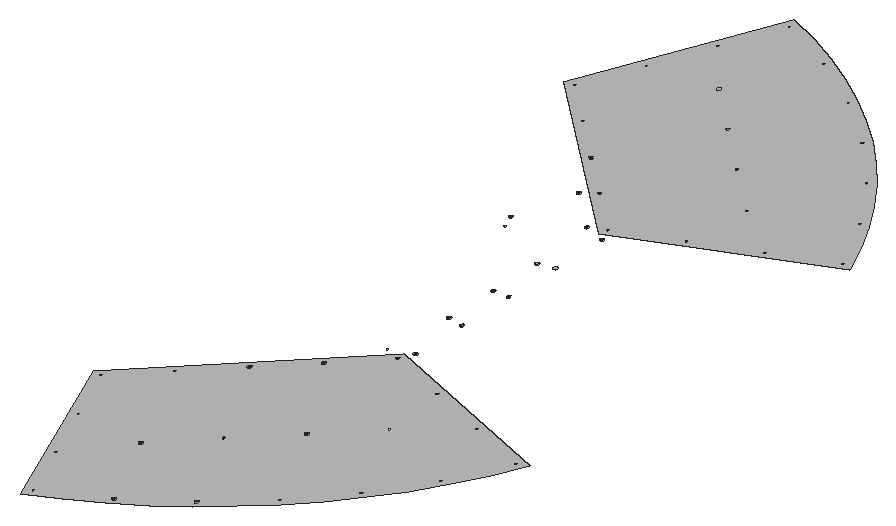
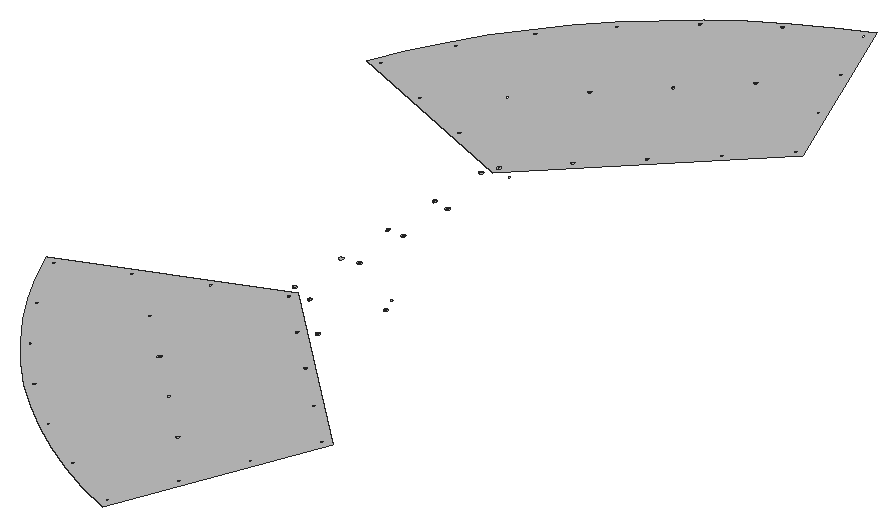
# SketchUp Ruby script. Lengths in inches.
U = 1.inch
M = Sketchup.active_model
def pt(a) = Geom::Point3d.new(a.map { |v| v * U })
def face(e, loops, mat)
  f = e.add_face(loops[0].map { |a| pt(a) })
  loops[1..].each { |l| e.add_face(l.map { |a| pt(a) }).erase! }
  f.material = f.back_material = mat if mat
  f
end
# faces: each face lists its corners as indices into pts; further lists are holes
def faces(e, pts, list, mat = nil) = list.each { |f| face(e, (f[0].is_a?(Array) ? f : [f]).map { |l| l.map { |i| pts[i] } }, mat) }
# xy, xz, yz: faces in a plane at the given z, y or x. An outline is a flat list of corners, or four numbers for a rectangle; further outlines are holes
def ring(l) = l.size == 4 ? [[l[0], l[1]], [l[2], l[1]], [l[2], l[3]], [l[0], l[3]]] : l.each_slice(2).to_a
def flat(e, list, mat, &to3) = list.each { |f| face(e, (f[0].is_a?(Array) ? f : [f]).map { |l| ring(l).map { |u, v| to3.(u, v) } }, mat) }
def xy(e, z, list, mat = nil) = flat(e, list, mat) { |x, y| [x, y, z] }
def xz(e, y, list, mat = nil) = flat(e, list, mat) { |x, z| [x, y, z] }
def yz(e, x, list, mat = nil) = flat(e, list, mat) { |y, z| [x, y, z] }
def lines(e, pts, list) = list.each { |a, b| e.add_line(pt(pts[a]), pt(pts[b])) }
# prism: a flat outline (further loops are holes) pulled along v
def prism(e, loops, v, mat = nil)
  f = face(e, loops, mat); d = Geom::Vector3d.new(v.map { |x| x * U })
  f.pushpull(f.normal.samedirection?(d) ? d.length : -d.length)
end
def box(e, o, s, mat = nil) = prism(e, [[o, [o[0] + s[0], o[1], o[2]], [o[0] + s[0], o[1] + s[1], o[2]], [o[0], o[1] + s[1], o[2]]]], [0, 0, s[2]], mat)
def at(x, y, z, deg = 0) = Geom::Transformation.translation(pt([x, y, z])) * Geom::Transformation.rotation(ORIGIN, Z_AXIS, deg.degrees)
def axes(o, x, y, z) = Geom::Transformation.new([*x, 0, *y, 0, *z, 0, *pt(o).to_a, 1])
def part(name) = M.definitions.add(name)
# library, detail: a bought-in or finely detailed component or shape, given as its bounding box
def library(name, o, s) = part(name).tap { |d| box(d.entities, o, s) }
def detail(e, o, s) = box(e.add_group.entities, o, s)
def put(e, d, t, mat = nil) = e.add_instance(d, t).tap { |i| i.material = mat if mat }
def group(e, t, mat = nil) = e.add_group.tap { |g| g.transformation = t; g.material = mat if mat }.entities
root = M.entities
M.materials.add("[Metal_Steel_Textured_White]").color = [191, 191, 191]
xy(root,3.625,[[[160.003,138.789,156.019,148.407,164.789,157.176,174.407,153.192,173.688,151.606,172.867,150.07,171.947,148.591,170.933,147.176,169.828,145.829,168.637,144.558,167.366,143.368,166.02,142.263,164.604,141.248,163.125,140.329,161.589,139.508],[162.784,154.518,162.807,154.521,162.829,154.53,162.847,154.545,162.861,154.563,162.87,154.584,162.873,154.607,162.87,154.63,162.861,154.652,162.847,154.67,162.829,154.684,162.807,154.693,162.784,154.696,162.761,154.693,162.74,154.684,162.721,154.67,162.707,154.652,162.698,154.63,162.695,154.607,162.698,154.584,162.707,154.563,162.721,154.545,162.74,154.53,162.761,154.521],[156.49,148.224,156.513,148.227,156.534,148.236,156.553,148.25,156.567,148.269,156.576,148.29,156.579,148.313,156.576,148.336,156.567,148.358,156.553,148.376,156.534,148.39,156.513,148.399,156.49,148.402,156.467,148.399,156.445,148.39,156.427,148.376,156.413,148.358,156.404,148.336,156.401,148.313,156.404,148.29,156.413,148.269,156.427,148.25,156.445,148.236,156.467,148.227],[168.355,144.751,168.378,144.755,168.399,144.763,168.418,144.778,168.432,144.796,168.441,144.817,168.444,144.84,168.441,144.863,168.432,144.885,168.418,144.903,168.399,144.917,168.378,144.926,168.355,144.929,168.332,144.926,168.31,144.917,168.292,144.903,168.278,144.885,168.269,144.863,168.266,144.84,168.269,144.817,168.278,144.796,168.292,144.778,168.31,144.763,168.332,144.755],[157.732,145.224,157.755,145.227,157.777,145.236,157.795,145.25,157.809,145.269,157.818,145.29,157.821,145.313,157.818,145.336,157.809,145.358,157.795,145.376,157.777,145.39,157.755,145.399,157.732,145.402,157.709,145.399,157.688,145.39,157.67,145.376,157.656,145.358,157.647,145.336,157.644,145.313,157.647,145.29,157.656,145.269,157.67,145.25,157.688,145.236,157.709,145.227],[158.588,150.322,158.611,150.325,158.632,150.334,158.651,150.348,158.665,150.367,158.674,150.388,158.677,150.411,158.674,150.434,158.665,150.456,158.651,150.474,158.632,150.488,158.611,150.497,158.588,150.5,158.565,150.497,158.544,150.488,158.525,150.474,158.511,150.456,158.502,150.434,158.499,150.411,158.502,150.388,158.511,150.367,158.525,150.348,158.544,150.334,158.565,150.325],[173.882,152.889,173.905,152.892,173.927,152.901,173.945,152.915,173.959,152.933,173.968,152.955,173.971,152.978,173.968,153.001,173.959,153.022,173.945,153.04,173.927,153.055,173.905,153.063,173.882,153.066,173.859,153.063,173.838,153.055,173.819,153.04,173.805,153.022,173.796,153.001,173.793,152.978,173.796,152.955,173.805,152.933,173.819,152.915,173.838,152.901,173.859,152.892],[163.155,140.72,163.178,140.723,163.2,140.732,163.218,140.746,163.232,140.764,163.241,140.786,163.244,140.809,163.241,140.832,163.232,140.853,163.218,140.871,163.2,140.886,163.178,140.894,163.155,140.897,163.132,140.894,163.111,140.886,163.093,140.871,163.078,140.853,163.07,140.832,163.066,140.809,163.07,140.786,163.078,140.764,163.093,140.746,163.111,140.732,163.132,140.723],[168.197,151.933,168.22,151.936,168.241,151.945,168.26,151.959,168.274,151.977,168.283,151.999,168.286,152.022,168.283,152.045,168.274,152.066,168.26,152.085,168.241,152.099,168.22,152.108,168.197,152.111,168.174,152.108,168.152,152.099,168.134,152.085,168.12,152.066,168.111,152.045,168.108,152.022,168.111,151.999,168.12,151.977,168.134,151.959,168.152,151.945,168.174,151.936],[170.882,154.131,170.905,154.134,170.927,154.143,170.945,154.157,170.959,154.176,170.968,154.197,170.971,154.22,170.968,154.243,170.959,154.265,170.945,154.283,170.927,154.297,170.905,154.306,170.882,154.309,170.859,154.306,170.838,154.297,170.819,154.283,170.805,154.265,170.796,154.243,170.793,154.22,170.796,154.197,170.805,154.176,170.819,154.157,170.838,154.143,170.859,154.134],[165.882,142.572,165.905,142.575,165.927,142.584,165.945,142.598,165.959,142.616,165.968,142.638,165.971,142.661,165.968,142.684,165.959,142.705,165.945,142.724,165.927,142.738,165.905,142.747,165.882,142.75,165.859,142.747,165.838,142.738,165.819,142.724,165.805,142.705,165.796,142.684,165.793,142.661,165.796,142.638,165.805,142.616,165.819,142.598,165.838,142.584,165.859,142.575],[167.882,155.374,167.905,155.377,167.927,155.386,167.945,155.4,167.959,155.418,167.968,155.44,167.971,155.463,167.968,155.486,167.959,155.507,167.945,155.526,167.927,155.54,167.905,155.549,167.882,155.552,167.859,155.549,167.838,155.54,167.819,155.526,167.805,155.507,167.796,155.486,167.793,155.463,167.796,155.44,167.805,155.418,167.819,155.4,167.838,155.386,167.859,155.377],[161.174,144.91,161.197,144.913,161.218,144.922,161.236,144.936,161.251,144.954,161.259,144.976,161.262,144.999,161.259,145.022,161.251,145.043,161.236,145.061,161.218,145.076,161.197,145.084,161.174,145.087,161.151,145.084,161.129,145.076,161.111,145.061,161.097,145.043,161.088,145.022,161.085,144.999,161.088,144.976,161.097,144.954,161.111,144.936,161.129,144.922,161.151,144.913],[165.856,149.592,165.879,149.595,165.9,149.604,165.919,149.618,165.933,149.636,165.942,149.658,165.945,149.681,165.942,149.704,165.933,149.725,165.919,149.744,165.9,149.758,165.879,149.767,165.856,149.77,165.833,149.767,165.811,149.758,165.793,149.744,165.779,149.725,165.77,149.704,165.767,149.681,165.77,149.658,165.779,149.636,165.793,149.618,165.811,149.604,165.833,149.595],[160.686,152.42,160.709,152.423,160.73,152.432,160.749,152.446,160.763,152.465,160.772,152.486,160.775,152.509,160.772,152.532,160.763,152.554,160.749,152.572,160.73,152.586,160.709,152.595,160.686,152.598,160.663,152.595,160.642,152.586,160.623,152.572,160.609,152.554,160.6,152.532,160.597,152.509,160.6,152.486,160.609,152.465,160.623,152.446,160.642,152.432,160.663,152.423],[172.387,149.951,172.41,149.954,172.431,149.963,172.45,149.977,172.464,149.995,172.473,150.017,172.476,150.04,172.473,150.063,172.464,150.084,172.45,150.103,172.431,150.117,172.41,150.126,172.387,150.129,172.364,150.126,172.342,150.117,172.324,150.103,172.31,150.084,172.301,150.063,172.298,150.04,172.301,150.017,172.31,149.995,172.324,149.977,172.342,149.963,172.364,149.954],[164.882,156.617,164.905,156.62,164.927,156.628,164.945,156.643,164.959,156.661,164.968,156.682,164.971,156.705,164.968,156.728,164.959,156.75,164.945,156.768,164.927,156.782,164.905,156.791,164.882,156.794,164.859,156.791,164.838,156.782,164.819,156.768,164.805,156.75,164.796,156.728,164.793,156.705,164.796,156.682,164.805,156.661,164.819,156.643,164.838,156.628,164.859,156.62],[158.975,142.224,158.998,142.227,159.02,142.236,159.038,142.25,159.052,142.269,159.061,142.29,159.064,142.313,159.061,142.336,159.052,142.358,159.038,142.376,159.02,142.39,158.998,142.399,158.975,142.402,158.952,142.399,158.931,142.39,158.912,142.376,158.898,142.358,158.889,142.336,158.886,142.313,158.889,142.29,158.898,142.269,158.912,142.25,158.931,142.236,158.952,142.227],[160.218,139.224,160.241,139.227,160.262,139.236,160.281,139.25,160.295,139.269,160.304,139.29,160.307,139.313,160.304,139.336,160.295,139.358,160.281,139.376,160.262,139.39,160.241,139.399,160.218,139.402,160.195,139.399,160.173,139.39,160.155,139.376,160.141,139.358,160.132,139.336,160.129,139.313,160.132,139.29,160.141,139.269,160.155,139.25,160.173,139.236,160.195,139.227],[163.515,147.251,163.538,147.254,163.559,147.263,163.577,147.277,163.592,147.295,163.6,147.317,163.604,147.34,163.6,147.363,163.592,147.384,163.577,147.402,163.559,147.417,163.538,147.425,163.515,147.429,163.492,147.425,163.47,147.417,163.452,147.402,163.4375,147.384,163.429,147.363,163.426,147.34,163.429,147.317,163.4375,147.295,163.452,147.277,163.47,147.263,163.492,147.254],[170.535,147.224,170.558,147.227,170.579,147.236,170.597,147.25,170.612,147.269,170.62,147.29,170.624,147.313,170.62,147.336,170.612,147.358,170.597,147.376,170.579,147.39,170.558,147.399,170.535,147.402,170.512,147.399,170.49,147.39,170.472,147.376,170.458,147.358,170.449,147.336,170.446,147.313,170.449,147.29,170.458,147.269,170.472,147.25,170.49,147.236,170.512,147.227]],[[163.155,140.72,163.132,140.723,163.111,140.732,163.093,140.746,163.078,140.764,163.07,140.786,163.066,140.809,163.07,140.832,163.078,140.853,163.093,140.871,163.111,140.886,163.132,140.894,163.155,140.897,163.178,140.894,163.2,140.886,163.218,140.871,163.232,140.853,163.241,140.832,163.244,140.809,163.241,140.786,163.232,140.764,163.218,140.746,163.2,140.732,163.178,140.723],[163.155,140.721,163.178,140.724,163.199,140.732,163.218,140.746,163.232,140.765,163.24,140.786,163.243,140.809,163.24,140.831,163.232,140.852,163.218,140.871,163.199,140.885,163.178,140.893,163.155,140.896,163.133,140.893,163.111,140.885,163.093,140.871,163.079,140.852,163.07,140.831,163.067,140.809,163.07,140.786,163.079,140.765,163.093,140.746,163.111,140.732,163.133,140.724]],[[163.155,140.721,163.133,140.724,163.111,140.732,163.093,140.746,163.079,140.765,163.07,140.786,163.067,140.809,163.07,140.831,163.079,140.852,163.093,140.871,163.111,140.885,163.133,140.893,163.155,140.896,163.178,140.893,163.199,140.885,163.218,140.871,163.232,140.852,163.24,140.831,163.243,140.809,163.24,140.786,163.232,140.765,163.218,140.746,163.199,140.732,163.178,140.724],[163.155,140.772,163.165,140.773,163.174,140.777,163.181,140.783,163.187,140.79,163.191,140.799,163.192,140.809,163.191,140.818,163.187,140.827,163.181,140.834,163.174,140.84,163.165,140.844,163.155,140.845,163.146,140.844,163.137,140.84,163.13,140.834,163.124,140.827,163.12,140.818,163.119,140.809,163.12,140.799,163.124,140.79,163.13,140.783,163.137,140.777,163.146,140.773]],[163.15,140.789,163.145,140.791,163.141,140.794,163.138,140.799,163.136,140.803,163.135,140.809,163.136,140.814,163.138,140.819,163.141,140.823,163.145,140.826,163.15,140.828,163.161,140.828,163.165,140.826,163.169,140.823,163.173,140.819,163.175,140.814,163.175,140.803,163.173,140.799,163.169,140.794,163.165,140.791,163.161,140.789],[[165.882,142.572,165.859,142.575,165.838,142.584,165.819,142.598,165.805,142.616,165.796,142.638,165.793,142.661,165.796,142.684,165.805,142.705,165.819,142.724,165.838,142.738,165.859,142.747,165.882,142.75,165.905,142.747,165.927,142.738,165.945,142.724,165.959,142.705,165.968,142.684,165.971,142.661,165.968,142.638,165.959,142.616,165.945,142.598,165.927,142.584,165.905,142.575],[165.882,142.573,165.905,142.576,165.926,142.585,165.944,142.599,165.958,142.617,165.967,142.638,165.97,142.661,165.967,142.683,165.958,142.705,165.944,142.723,165.926,142.737,165.905,142.746,165.882,142.749,165.859,142.746,165.838,142.737,165.82,142.723,165.806,142.705,165.797,142.683,165.794,142.661,165.797,142.638,165.806,142.617,165.82,142.599,165.838,142.585,165.859,142.576]],
  [[165.882,142.573,165.859,142.576,165.838,142.585,165.82,142.599,165.806,142.617,165.797,142.638,165.794,142.661,165.797,142.683,165.806,142.705,165.82,142.723,165.838,142.737,165.859,142.746,165.882,142.749,165.905,142.746,165.926,142.737,165.944,142.723,165.958,142.705,165.967,142.683,165.97,142.661,165.967,142.638,165.958,142.617,165.944,142.599,165.926,142.585,165.905,142.576],[165.882,142.624,165.892,142.625,165.9,142.629,165.908,142.635,165.914,142.642,165.917,142.651,165.919,142.661,165.917,142.67,165.914,142.679,165.908,142.687,165.9,142.692,165.892,142.696,165.882,142.697,165.873,142.696,165.864,142.692,165.856,142.687,165.85,142.679,165.847,142.67,165.846,142.661,165.847,142.651,165.85,142.642,165.856,142.635,165.864,142.629,165.873,142.625]],[[161.174,144.91,161.151,144.913,161.129,144.922,161.111,144.936,161.097,144.954,161.088,144.976,161.085,144.999,161.088,145.022,161.097,145.043,161.111,145.061,161.129,145.076,161.151,145.084,161.174,145.087,161.197,145.084,161.218,145.076,161.236,145.061,161.251,145.043,161.259,145.022,161.262,144.999,161.259,144.976,161.251,144.954,161.236,144.936,161.218,144.922,161.197,144.913],[161.174,144.911,161.196,144.914,161.218,144.922,161.236,144.936,161.25,144.955,161.258,144.976,161.261,144.999,161.258,145.021,161.25,145.043,161.236,145.061,161.218,145.075,161.196,145.083,161.174,145.086,161.151,145.083,161.13,145.075,161.111,145.061,161.097,145.043,161.089,145.021,161.086,144.999,161.089,144.976,161.097,144.955,161.111,144.936,161.13,144.922,161.151,144.914]],[[163.515,147.251,163.492,147.254,163.47,147.263,163.452,147.277,163.4375,147.295,163.429,147.317,163.426,147.34,163.429,147.363,163.4375,147.384,163.452,147.402,163.47,147.417,163.492,147.425,163.515,147.429,163.538,147.425,163.559,147.417,163.577,147.402,163.592,147.384,163.6,147.363,163.604,147.34,163.6,147.317,163.592,147.295,163.577,147.277,163.559,147.263,163.538,147.254],[163.515,147.252,163.537,147.255,163.559,147.263,163.577,147.277,163.591,147.296,163.6,147.317,163.603,147.34,163.6,147.362,163.591,147.384,163.577,147.402,163.559,147.416,163.537,147.425,163.515,147.428,163.492,147.425,163.471,147.416,163.452,147.402,163.438,147.384,163.43,147.362,163.427,147.34,163.43,147.317,163.438,147.296,163.452,147.277,163.471,147.263,163.492,147.255]],[[163.515,147.303,163.505,147.304,163.496,147.308,163.489,147.314,163.483,147.321,163.479,147.33,163.478,147.34,163.479,147.349,163.483,147.358,163.489,147.365,163.496,147.371,163.505,147.375,163.515,147.376,163.524,147.375,163.533,147.371,163.541,147.365,163.546,147.358,163.55,147.349,163.551,147.34,163.55,147.33,163.546,147.321,163.541,147.314,163.533,147.308,163.524,147.304],[163.509,147.32,163.52,147.32,163.525,147.322,163.529,147.326,163.532,147.33,163.534,147.334,163.535,147.34,163.534,147.345,163.532,147.35,163.529,147.354,163.525,147.357,163.52,147.359,163.515,147.36,163.509,147.359,163.505,147.357,163.501,147.354,163.497,147.35,163.495,147.345,163.495,147.334,163.497,147.33,163.505,147.322]],[163.509,147.32,163.505,147.322,163.497,147.33,163.495,147.334,163.495,147.345,163.497,147.35,163.501,147.354,163.505,147.357,163.509,147.359,163.515,147.36,163.52,147.359,163.525,147.357,163.529,147.354,163.532,147.35,163.534,147.345,163.535,147.34,163.534,147.334,163.532,147.33,163.529,147.326,163.525,147.322,163.52,147.32],
  [[165.856,149.592,165.833,149.595,165.811,149.604,165.793,149.618,165.779,149.636,165.77,149.658,165.767,149.681,165.77,149.704,165.779,149.725,165.793,149.744,165.811,149.758,165.833,149.767,165.856,149.77,165.879,149.767,165.9,149.758,165.919,149.744,165.933,149.725,165.942,149.704,165.945,149.681,165.942,149.658,165.933,149.636,165.919,149.618,165.9,149.604,165.879,149.595],[165.856,149.593,165.878,149.596,165.9,149.605,165.918,149.619,165.932,149.637,165.941,149.658,165.944,149.681,165.941,149.703,165.932,149.725,165.918,149.743,165.9,149.757,165.878,149.766,165.856,149.769,165.833,149.766,165.812,149.757,165.794,149.743,165.78,149.725,165.771,149.703,165.768,149.681,165.771,149.658,165.78,149.637,165.794,149.619,165.812,149.605,165.833,149.596]],[[160.686,152.42,160.663,152.423,160.642,152.432,160.623,152.446,160.609,152.465,160.6,152.486,160.597,152.509,160.6,152.532,160.609,152.554,160.623,152.572,160.642,152.586,160.663,152.595,160.686,152.598,160.709,152.595,160.73,152.586,160.749,152.572,160.763,152.554,160.772,152.532,160.775,152.509,160.772,152.486,160.763,152.465,160.749,152.446,160.73,152.432,160.709,152.423],[160.686,152.421,160.709,152.424,160.73,152.433,160.748,152.447,160.762,152.465,160.771,152.487,160.774,152.509,160.771,152.532,160.762,152.553,160.748,152.571,160.73,152.585,160.709,152.594,160.686,152.597,160.663,152.594,160.642,152.585,160.624,152.571,160.61,152.553,160.601,152.532,160.598,152.509,160.601,152.487,160.61,152.465,160.624,152.447,160.642,152.433,160.663,152.424]],[[160.686,152.473,160.677,152.474,160.668,152.478,160.66,152.483,160.654,152.491,160.651,152.5,160.649,152.509,160.651,152.519,160.654,152.528,160.66,152.535,160.668,152.541,160.677,152.545,160.686,152.546,160.696,152.545,160.704,152.541,160.712,152.535,160.718,152.528,160.721,152.519,160.723,152.509,160.721,152.5,160.718,152.491,160.712,152.483,160.704,152.478,160.696,152.474],[160.686,152.489,160.691,152.49,160.696,152.492,160.7,152.495,160.703,152.499,160.705,152.504,160.706,152.509,160.705,152.514,160.703,152.519,160.7,152.523,160.696,152.527,160.691,152.529,160.681,152.529,160.676,152.527,160.672,152.523,160.669,152.519,160.667,152.514,160.666,152.509,160.667,152.504,160.669,152.499,160.672,152.495,160.676,152.492,160.681,152.49]],[160.686,152.489,160.681,152.49,160.676,152.492,160.672,152.495,160.669,152.499,160.667,152.504,160.666,152.509,160.667,152.514,160.669,152.519,160.672,152.523,160.676,152.527,160.681,152.529,160.691,152.529,160.696,152.527,160.7,152.523,160.703,152.519,160.705,152.514,160.706,152.509,160.705,152.504,160.703,152.499,160.7,152.495,160.696,152.492,160.691,152.49],[[162.784,154.518,162.761,154.521,162.74,154.53,162.721,154.545,162.707,154.563,162.698,154.584,162.695,154.607,162.698,154.63,162.707,154.652,162.721,154.67,162.74,154.684,162.761,154.693,162.784,154.696,162.807,154.693,162.829,154.684,162.847,154.67,162.861,154.652,162.87,154.63,162.873,154.607,162.87,154.584,162.861,154.563,162.847,154.545,162.829,154.53,162.807,154.521],[162.784,154.519,162.807,154.522,162.828,154.531,162.846,154.545,162.86,154.563,162.869,154.585,162.872,154.607,162.869,154.63,162.86,154.651,162.846,154.67,162.828,154.684,162.807,154.692,162.784,154.695,162.761,154.692,162.74,154.684,162.722,154.67,162.708,154.651,162.699,154.63,162.696,154.607,162.699,154.585,162.708,154.563,162.722,154.545,162.74,154.531,162.761,154.522]],
  [[162.784,154.519,162.761,154.522,162.74,154.531,162.722,154.545,162.708,154.563,162.699,154.585,162.696,154.607,162.699,154.63,162.708,154.651,162.722,154.67,162.74,154.684,162.761,154.692,162.784,154.695,162.807,154.692,162.828,154.684,162.846,154.67,162.86,154.651,162.869,154.63,162.872,154.607,162.869,154.585,162.86,154.563,162.846,154.545,162.828,154.531,162.807,154.522],[162.784,154.571,162.794,154.572,162.802,154.576,162.81,154.581,162.816,154.589,162.819,154.598,162.821,154.607,162.819,154.617,162.816,154.626,162.81,154.633,162.802,154.639,162.794,154.643,162.784,154.644,162.775,154.643,162.766,154.639,162.758,154.633,162.752,154.626,162.749,154.617,162.748,154.607,162.749,154.598,162.752,154.589,162.758,154.581,162.766,154.576,162.775,154.572]],[[167.882,155.426,167.873,155.427,167.864,155.431,167.856,155.437,167.851,155.445,167.847,155.453,167.846,155.463,167.847,155.472,167.851,155.481,167.856,155.489,167.864,155.495,167.873,155.498,167.882,155.499,167.892,155.498,167.901,155.495,167.908,155.489,167.914,155.481,167.918,155.472,167.919,155.463,167.918,155.453,167.914,155.445,167.908,155.437,167.901,155.431,167.892,155.427],[167.882,155.443,167.887,155.444,167.892,155.446,167.896,155.449,167.899,155.453,167.901,155.458,167.902,155.463,167.901,155.468,167.899,155.473,167.896,155.477,167.892,155.48,167.887,155.482,167.882,155.483,167.877,155.482,167.872,155.48,167.868,155.477,167.865,155.473,167.863,155.468,167.862,155.463,167.863,155.458,167.865,155.453,167.868,155.449,167.872,155.446,167.877,155.444]],[167.882,155.443,167.877,155.444,167.872,155.446,167.868,155.449,167.865,155.453,167.863,155.458,167.862,155.463,167.863,155.468,167.865,155.473,167.868,155.477,167.872,155.48,167.877,155.482,167.882,155.483,167.887,155.482,167.892,155.48,167.896,155.477,167.899,155.473,167.901,155.468,167.902,155.463,167.901,155.458,167.899,155.453,167.896,155.449,167.892,155.446,167.887,155.444],[[164.882,156.618,164.859,156.621,164.838,156.629,164.82,156.643,164.806,156.661,164.797,156.683,164.794,156.705,164.797,156.728,164.806,156.749,164.82,156.768,164.838,156.782,164.859,156.79,164.882,156.793,164.905,156.79,164.926,156.782,164.944,156.768,164.958,156.749,164.967,156.728,164.97,156.705,164.967,156.683,164.958,156.661,164.944,156.643,164.926,156.629,164.905,156.621],[164.882,156.669,164.892,156.67,164.901,156.674,164.908,156.68,164.914,156.687,164.918,156.696,164.919,156.705,164.918,156.715,164.914,156.724,164.908,156.731,164.901,156.737,164.892,156.741,164.882,156.742,164.873,156.741,164.864,156.737,164.856,156.731,164.851,156.724,164.847,156.715,164.846,156.705,164.847,156.696,164.851,156.687,164.856,156.68,164.864,156.674,164.873,156.67]],[164.882,156.685,164.877,156.686,164.872,156.688,164.868,156.691,164.865,156.695,164.863,156.7,164.862,156.705,164.863,156.711,164.865,156.715,164.868,156.72,164.872,156.723,164.877,156.725,164.887,156.725,164.892,156.723,164.896,156.72,164.9,156.715,164.902,156.711,164.902,156.7,164.9,156.695,164.896,156.691,164.892,156.688,164.887,156.686],
  [164.084,157.016,164.079,157.017,164.074,157.019,164.07,157.022,164.067,157.026,164.065,157.031,164.064,157.036,164.065,157.041,164.067,157.046,164.07,157.05,164.074,157.053,164.079,157.055,164.084,157.056,164.089,157.055,164.094,157.053,164.098,157.05,164.101,157.046,164.103,157.041,164.104,157.036,164.103,157.031,164.101,157.026,164.098,157.022,164.094,157.019,164.089,157.017],[[165.188,157.354,165.165,157.357,165.143,157.366,165.125,157.38,165.111,157.399,165.102,157.42,165.099,157.443,165.102,157.466,165.111,157.488,165.125,157.506,165.143,157.52,165.165,157.529,165.188,157.532,165.211,157.529,165.232,157.52,165.251,157.506,165.265,157.488,165.274,157.466,165.277,157.443,165.274,157.42,165.265,157.399,165.251,157.38,165.232,157.366,165.211,157.357],[165.188,157.355,165.211,157.358,165.232,157.367,165.25,157.381,165.264,157.399,165.273,157.42,165.276,157.443,165.273,157.466,165.264,157.487,165.25,157.505,165.232,157.519,165.211,157.528,165.188,157.531,165.165,157.528,165.144,157.519,165.126,157.505,165.112,157.487,165.103,157.466,165.1,157.443,165.103,157.42,165.112,157.399,165.126,157.381,165.144,157.367,165.165,157.358]],[[165.188,157.355,165.165,157.358,165.144,157.367,165.126,157.381,165.112,157.399,165.103,157.42,165.1,157.443,165.103,157.466,165.112,157.487,165.126,157.505,165.144,157.519,165.165,157.528,165.188,157.531,165.211,157.528,165.232,157.519,165.25,157.505,165.264,157.487,165.273,157.466,165.276,157.443,165.273,157.42,165.264,157.399,165.25,157.381,165.232,157.367,165.211,157.358],[165.188,157.407,165.197,157.408,165.206,157.411,165.214,157.417,165.219,157.425,165.223,157.434,165.224,157.443,165.223,157.453,165.219,157.461,165.214,157.469,165.206,157.475,165.197,157.478,165.188,157.48,165.178,157.478,165.169,157.475,165.162,157.469,165.156,157.461,165.152,157.453,165.151,157.443,165.152,157.434,165.156,157.425,165.162,157.417,165.169,157.411,165.178,157.408]],[[165.188,160.321,165.165,160.324,165.143,160.333,165.125,160.347,165.111,160.366,165.102,160.387,165.099,160.41,165.102,160.433,165.111,160.455,165.125,160.473,165.143,160.487,165.165,160.496,165.188,160.499,165.211,160.496,165.232,160.487,165.251,160.473,165.265,160.455,165.274,160.433,165.277,160.41,165.274,160.387,165.265,160.366,165.251,160.347,165.232,160.333,165.211,160.324],[165.188,160.322,165.211,160.325,165.232,160.334,165.25,160.348,165.264,160.366,165.273,160.388,165.276,160.41,165.273,160.433,165.264,160.454,165.25,160.472,165.232,160.486,165.211,160.495,165.188,160.498,165.165,160.495,165.144,160.486,165.126,160.472,165.112,160.454,165.103,160.433,165.1,160.41,165.103,160.388,165.112,160.366,165.126,160.348,165.144,160.334,165.165,160.325]],[[165.188,160.374,165.178,160.375,165.169,160.379,165.162,160.384,165.156,160.392,165.152,160.401,165.151,160.41,165.152,160.42,165.156,160.429,165.162,160.436,165.169,160.442,165.178,160.446,165.188,160.447,165.197,160.446,165.206,160.442,165.214,160.436,165.219,160.429,165.223,160.42,165.224,160.41,165.223,160.401,165.219,160.392,165.214,160.384,165.206,160.379,165.197,160.375],[165.188,160.39,165.193,160.391,165.198,160.393,165.202,160.396,165.205,160.4,165.207,160.405,165.208,160.41,165.207,160.415,165.205,160.42,165.202,160.424,165.198,160.428,165.193,160.43,165.183,160.43,165.178,160.428,165.174,160.424,165.171,160.42,165.169,160.415,165.168,160.41,165.169,160.405,165.171,160.4,165.174,160.396,165.178,160.393,165.183,160.391]],
  [165.188,160.39,165.183,160.391,165.178,160.393,165.174,160.396,165.171,160.4,165.169,160.405,165.168,160.41,165.169,160.415,165.171,160.42,165.174,160.424,165.178,160.428,165.183,160.43,165.193,160.43,165.198,160.428,165.202,160.424,165.205,160.42,165.207,160.415,165.208,160.41,165.207,160.405,165.205,160.4,165.202,160.396,165.198,160.393,165.193,160.391],[[164.389,160.487,164.366,160.49,164.345,160.499,164.327,160.513,164.3125,160.531,164.303,160.553,164.3,160.576,164.303,160.599,164.3125,160.62,164.327,160.638,164.345,160.653,164.366,160.661,164.389,160.665,164.412,160.661,164.434,160.653,164.452,160.638,164.466,160.62,164.475,160.599,164.478,160.576,164.475,160.553,164.466,160.531,164.452,160.513,164.434,160.499,164.412,160.49],[164.389,160.488,164.412,160.491,164.433,160.499,164.452,160.513,164.466,160.532,164.474,160.553,164.477,160.576,164.474,160.598,164.466,160.62,164.452,160.638,164.433,160.652,164.412,160.661,164.389,160.664,164.367,160.661,164.345,160.652,164.327,160.638,164.313,160.62,164.304,160.598,164.301,160.576,164.304,160.553,164.313,160.532,164.327,160.513,164.345,160.499,164.367,160.491]],[[164.389,160.539,164.38,160.54,164.371,160.544,164.363,160.55,164.358,160.557,164.354,160.566,164.353,160.576,164.354,160.585,164.358,160.594,164.363,160.602,164.371,160.607,164.38,160.611,164.389,160.612,164.399,160.611,164.408,160.607,164.415,160.602,164.421,160.594,164.425,160.585,164.426,160.576,164.425,160.566,164.421,160.557,164.415,160.55,164.408,160.544,164.399,160.54],[164.384,160.556,164.395,160.556,164.399,160.558,164.407,160.566,164.409,160.57,164.409,160.581,164.407,160.586,164.403,160.59,164.399,160.593,164.395,160.595,164.389,160.596,164.384,160.595,164.379,160.593,164.375,160.59,164.372,160.586,164.37,160.581,164.369,160.576,164.37,160.57,164.372,160.566,164.375,160.562,164.379,160.558]],[164.384,160.556,164.379,160.558,164.375,160.562,164.372,160.566,164.37,160.57,164.369,160.576,164.37,160.581,164.372,160.586,164.375,160.59,164.379,160.593,164.384,160.595,164.389,160.596,164.395,160.595,164.399,160.593,164.403,160.59,164.407,160.586,164.409,160.581,164.409,160.57,164.407,160.566,164.399,160.558,164.395,160.556],[164.389,163.289,164.366,163.292,164.345,163.3,164.327,163.315,164.3125,163.333,164.303,163.354,164.3,163.377,164.301,163.377,164.304,163.355,164.313,163.333,164.327,163.315,164.345,163.301,164.367,163.292,164.389,163.289,164.412,163.292,164.433,163.301,164.452,163.315,164.466,163.333,164.474,163.355,164.477,163.377,164.478,163.377,164.475,163.354,164.466,163.333,164.452,163.315,164.434,163.3,164.412,163.292],
  [165.188,163.289,165.165,163.292,165.143,163.3,165.125,163.315,165.111,163.333,165.102,163.354,165.099,163.377,165.1,163.377,165.103,163.355,165.112,163.333,165.126,163.315,165.144,163.301,165.165,163.292,165.188,163.289,165.211,163.292,165.232,163.301,165.25,163.315,165.264,163.333,165.273,163.355,165.276,163.377,165.277,163.377,165.274,163.354,165.265,163.333,165.251,163.315,165.232,163.3,165.211,163.292],[164.389,163.341,164.38,163.342,164.371,163.346,164.363,163.352,164.358,163.359,164.354,163.368,164.353,163.377,164.369,163.377,164.37,163.372,164.372,163.367,164.375,163.363,164.379,163.36,164.384,163.358,164.389,163.357,164.395,163.358,164.399,163.36,164.403,163.363,164.407,163.367,164.409,163.372,164.409,163.377,164.426,163.377,164.425,163.368,164.421,163.359,164.415,163.352,164.408,163.346,164.399,163.342],[165.188,163.341,165.178,163.342,165.169,163.346,165.162,163.352,165.156,163.359,165.152,163.368,165.151,163.377,165.168,163.377,165.169,163.372,165.171,163.367,165.174,163.363,165.178,163.36,165.183,163.358,165.188,163.357,165.193,163.358,165.198,163.36,165.202,163.363,165.205,163.367,165.207,163.372,165.208,163.377,165.224,163.377,165.223,163.368,165.219,163.359,165.214,163.352,165.206,163.346,165.197,163.342],[165.188,163.357,165.183,163.358,165.178,163.36,165.174,163.363,165.171,163.367,165.169,163.372,165.168,163.377,165.208,163.377,165.207,163.372,165.205,163.367,165.202,163.363,165.198,163.36,165.193,163.358],[164.301,163.377,164.304,163.4,164.313,163.421,164.327,163.44,164.345,163.454,164.367,163.462,164.389,163.465,164.412,163.462,164.433,163.454,164.452,163.44,164.466,163.421,164.474,163.4,164.477,163.377,164.426,163.377,164.425,163.387,164.421,163.396,164.415,163.403,164.408,163.409,164.399,163.413,164.389,163.414,164.38,163.413,164.371,163.409,164.363,163.403,164.358,163.396,164.354,163.387,164.353,163.377],
  [164.353,163.377,164.354,163.387,164.358,163.396,164.363,163.403,164.371,163.409,164.38,163.413,164.389,163.414,164.399,163.413,164.408,163.409,164.415,163.403,164.421,163.396,164.425,163.387,164.426,163.377,164.409,163.377,164.409,163.383,164.407,163.387,164.403,163.392,164.399,163.395,164.395,163.397,164.384,163.397,164.379,163.395,164.375,163.392,164.372,163.387,164.37,163.383,164.369,163.377],[165.099,163.377,165.102,163.4,165.111,163.422,165.125,163.44,165.143,163.454,165.165,163.463,165.188,163.466,165.211,163.463,165.232,163.454,165.251,163.44,165.265,163.422,165.274,163.4,165.277,163.377,165.276,163.377,165.273,163.4,165.264,163.421,165.25,163.44,165.232,163.454,165.211,163.462,165.188,163.465,165.165,163.462,165.144,163.454,165.126,163.44,165.112,163.421,165.103,163.4,165.1,163.377],[165.151,163.377,165.152,163.387,165.156,163.396,165.162,163.403,165.169,163.409,165.178,163.413,165.188,163.414,165.197,163.413,165.206,163.409,165.214,163.403,165.219,163.396,165.223,163.387,165.224,163.377,165.208,163.377,165.207,163.383,165.205,163.387,165.202,163.392,165.198,163.395,165.193,163.397,165.183,163.397,165.178,163.395,165.174,163.392,165.171,163.387,165.169,163.383,165.168,163.377],[165.168,163.377,165.169,163.383,165.171,163.387,165.174,163.392,165.178,163.395,165.183,163.397,165.193,163.397,165.198,163.395,165.202,163.392,165.205,163.387,165.207,163.383,165.208,163.377],[[164.389,166.09,164.366,166.093,164.345,166.102,164.327,166.116,164.3125,166.135,164.303,166.156,164.3,166.179,164.303,166.202,164.3125,166.224,164.327,166.242,164.345,166.256,164.366,166.265,164.389,166.268,164.412,166.265,164.434,166.256,164.452,166.242,164.466,166.224,164.475,166.202,164.478,166.179,164.475,166.156,164.466,166.135,164.452,166.116,164.434,166.102,164.412,166.093],[164.389,166.091,164.412,166.094,164.433,166.103,164.452,166.117,164.466,166.135,164.474,166.156,164.477,166.179,164.474,166.202,164.466,166.223,164.452,166.241,164.433,166.255,164.412,166.264,164.389,166.267,164.367,166.264,164.345,166.255,164.327,166.241,164.313,166.223,164.304,166.202,164.301,166.179,164.304,166.156,164.313,166.135,164.327,166.117,164.345,166.103,164.367,166.094]],
  [[164.389,166.143,164.38,166.144,164.371,166.148,164.363,166.153,164.358,166.161,164.354,166.17,164.353,166.179,164.354,166.189,164.358,166.198,164.363,166.205,164.371,166.211,164.38,166.215,164.389,166.216,164.399,166.215,164.408,166.211,164.415,166.205,164.421,166.198,164.425,166.189,164.426,166.179,164.425,166.17,164.421,166.161,164.415,166.153,164.408,166.148,164.399,166.144],[164.389,166.159,164.395,166.16,164.399,166.162,164.403,166.165,164.407,166.169,164.409,166.174,164.409,166.184,164.407,166.189,164.399,166.197,164.395,166.198,164.389,166.199,164.379,166.197,164.375,166.193,164.372,166.189,164.37,166.184,164.369,166.179,164.37,166.174,164.372,166.169,164.375,166.165,164.379,166.162,164.384,166.16]],[[165.188,166.257,165.165,166.26,165.144,166.268,165.126,166.282,165.112,166.301,165.103,166.322,165.1,166.345,165.103,166.367,165.112,166.389,165.126,166.407,165.144,166.421,165.165,166.43,165.188,166.433,165.211,166.43,165.232,166.421,165.25,166.407,165.264,166.389,165.273,166.367,165.276,166.345,165.273,166.322,165.264,166.301,165.25,166.282,165.232,166.268,165.211,166.26],[165.188,166.308,165.197,166.309,165.206,166.313,165.214,166.319,165.219,166.326,165.223,166.335,165.224,166.345,165.223,166.354,165.219,166.363,165.214,166.37,165.206,166.376,165.197,166.38,165.188,166.381,165.178,166.38,165.169,166.376,165.162,166.37,165.156,166.363,165.152,166.354,165.151,166.345,165.152,166.335,165.156,166.326,165.162,166.319,165.169,166.313,165.178,166.309]],[[161.486,167.742,161.476,167.743,161.467,167.747,161.46,167.752,161.454,167.76,161.45,167.769,161.449,167.778,161.45,167.788,161.454,167.797,161.46,167.804,161.467,167.81,161.476,167.814,161.486,167.815,161.495,167.814,161.504,167.81,161.511,167.804,161.517,167.797,161.521,167.788,161.522,167.778,161.521,167.769,161.517,167.76,161.511,167.752,161.504,167.747,161.495,167.743],[161.486,167.758,161.491,167.759,161.496,167.761,161.5,167.764,161.503,167.768,161.505,167.773,161.506,167.778,161.505,167.783,161.503,167.788,161.5,167.792,161.496,167.796,161.491,167.798,161.48,167.798,161.476,167.796,161.471,167.792,161.468,167.788,161.466,167.783,161.466,167.773,161.468,167.768,161.471,167.764,161.476,167.761,161.48,167.759]],[[161.18,168.427,161.157,168.43,161.136,168.439,161.117,168.453,161.103,168.471,161.094,168.493,161.091,168.516,161.094,168.539,161.103,168.56,161.117,168.579,161.136,168.593,161.157,168.602,161.18,168.605,161.203,168.602,161.224,168.593,161.243,168.579,161.257,168.56,161.266,168.539,161.269,168.516,161.266,168.493,161.257,168.471,161.243,168.453,161.224,168.439,161.203,168.43],[161.18,168.428,161.203,168.431,161.224,168.44,161.242,168.454,161.256,168.472,161.265,168.493,161.268,168.516,161.265,168.539,161.256,168.56,161.242,168.578,161.224,168.592,161.203,168.601,161.18,168.604,161.157,168.601,161.136,168.592,161.118,168.578,161.104,168.56,161.095,168.539,161.092,168.516,161.095,168.493,161.104,168.472,161.118,168.454,161.136,168.44,161.157,168.431]],[[161.18,168.479,161.171,168.481,161.162,168.484,161.154,168.49,161.148,168.498,161.145,168.506,161.143,168.516,161.145,168.525,161.148,168.534,161.154,168.542,161.162,168.548,161.171,168.551,161.18,168.552,161.189,168.551,161.198,168.548,161.206,168.542,161.212,168.534,161.215,168.525,161.217,168.516,161.215,168.506,161.212,168.498,161.206,168.49,161.198,168.484,161.189,168.481],[161.18,168.496,161.185,168.497,161.19,168.499,161.194,168.502,161.197,168.506,161.199,168.511,161.2,168.516,161.199,168.521,161.197,168.526,161.194,168.53,161.19,168.533,161.185,168.535,161.18,168.536,161.175,168.535,161.17,168.533,161.166,168.53,161.163,168.526,161.161,168.521,161.16,168.516,161.161,168.511,161.163,168.506,161.166,168.502,161.17,168.499,161.175,168.497]],
  [161.18,168.496,161.175,168.497,161.17,168.499,161.166,168.502,161.163,168.506,161.161,168.511,161.16,168.516,161.161,168.521,161.163,168.526,161.166,168.53,161.17,168.533,161.175,168.535,161.18,168.536,161.185,168.535,161.19,168.533,161.194,168.53,161.197,168.526,161.199,168.521,161.2,168.516,161.199,168.511,161.197,168.506,161.194,168.502,161.19,168.499,161.185,168.497],[[165.188,169.223,165.165,169.226,165.143,169.235,165.125,169.249,165.111,169.267,165.102,169.289,165.099,169.312,165.102,169.335,165.111,169.356,165.125,169.375,165.143,169.389,165.165,169.398,165.188,169.401,165.211,169.398,165.232,169.389,165.251,169.375,165.265,169.356,165.274,169.335,165.277,169.312,165.274,169.289,165.265,169.267,165.251,169.249,165.232,169.235,165.211,169.226],[165.188,169.224,165.211,169.227,165.232,169.236,165.25,169.25,165.264,169.268,165.273,169.289,165.276,169.312,165.273,169.334,165.264,169.356,165.25,169.374,165.232,169.388,165.211,169.397,165.188,169.4,165.165,169.397,165.144,169.388,165.126,169.374,165.112,169.356,165.103,169.334,165.1,169.312,165.103,169.289,165.112,169.268,165.126,169.25,165.144,169.236,165.165,169.227]],[[165.188,169.224,165.165,169.227,165.144,169.236,165.126,169.25,165.112,169.268,165.103,169.289,165.1,169.312,165.103,169.334,165.112,169.356,165.126,169.374,165.144,169.388,165.165,169.397,165.188,169.4,165.211,169.397,165.232,169.388,165.25,169.374,165.264,169.356,165.273,169.334,165.276,169.312,165.273,169.289,165.264,169.268,165.25,169.25,165.232,169.236,165.211,169.227],[165.188,169.275,165.197,169.276,165.206,169.28,165.214,169.286,165.219,169.293,165.223,169.302,165.224,169.312,165.223,169.321,165.219,169.33,165.214,169.338,165.206,169.343,165.197,169.347,165.188,169.348,165.178,169.347,165.169,169.343,165.162,169.338,165.156,169.33,165.152,169.321,165.151,169.312,165.152,169.302,165.156,169.293,165.162,169.286,165.169,169.28,165.178,169.276]],[[164.789,169.578,156.019,178.348,160.003,187.966,161.589,187.247,163.125,186.426,164.604,185.507,166.02,184.492,167.366,183.387,168.637,182.197,169.828,180.926,170.933,179.579,171.947,178.164,172.867,176.685,173.688,175.149,174.407,173.5625],[157.732,181.353,157.755,181.356,157.777,181.365,157.795,181.379,157.809,181.397,157.818,181.419,157.821,181.442,157.818,181.465,157.809,181.486,157.795,181.505,157.777,181.519,157.755,181.528,157.732,181.531,157.709,181.528,157.688,181.519,157.67,181.505,157.656,181.486,157.647,181.465,157.644,181.442,157.647,181.419,157.656,181.397,157.67,181.379,157.688,181.365,157.709,181.356],[163.515,179.326,163.538,179.329,163.559,179.338,163.577,179.352,163.592,179.371,163.6,179.392,163.604,179.415,163.6,179.438,163.592,179.46,163.577,179.478,163.559,179.492,163.538,179.501,163.515,179.504,163.492,179.501,163.47,179.492,163.452,179.478,163.4375,179.46,163.429,179.438,163.426,179.415,163.429,179.392,163.4375,179.371,163.452,179.352,163.47,179.338,163.492,179.329],[162.784,172.059,162.807,172.062,162.829,172.071,162.847,172.085,162.861,172.103,162.87,172.124,162.873,172.147,162.87,172.17,162.861,172.192,162.847,172.21,162.829,172.224,162.807,172.233,162.784,172.236,162.761,172.233,162.74,172.224,162.721,172.21,162.707,172.192,162.698,172.17,162.695,172.147,162.698,172.124,162.707,172.103,162.721,172.085,162.74,172.071,162.761,172.062],[173.882,173.688,173.905,173.691,173.927,173.7,173.945,173.714,173.959,173.733,173.968,173.754,173.971,173.777,173.968,173.8,173.959,173.822,173.945,173.84,173.927,173.854,173.905,173.863,173.882,173.866,173.859,173.863,173.838,173.854,173.819,173.84,173.805,173.822,173.796,173.8,173.793,173.777,173.796,173.754,173.805,173.733,173.819,173.714,173.838,173.7,173.859,173.691],[161.174,181.667,161.197,181.67,161.218,181.679,161.236,181.693,161.251,181.712,161.259,181.733,161.262,181.756,161.259,181.779,161.251,181.801,161.236,181.819,161.218,181.833,161.197,181.842,161.174,181.845,161.151,181.842,161.129,181.833,161.111,181.819,161.097,181.801,161.088,181.779,161.085,181.756,161.088,181.733,161.097,181.712,161.111,181.693,161.129,181.679,161.151,181.67],[158.588,176.255,158.611,176.258,158.632,176.267,158.651,176.281,158.665,176.299,158.674,176.321,158.677,176.344,158.674,176.367,158.665,176.388,158.651,176.407,158.632,176.421,158.611,176.43,158.588,176.433,158.565,176.43,158.544,176.421,158.525,176.407,158.511,176.388,158.502,176.367,158.499,176.344,158.502,176.321,158.511,176.299,158.525,176.281,158.544,176.267,158.565,176.258],[168.197,174.644,168.22,174.647,168.241,174.656,168.26,174.67,168.274,174.689,168.283,174.71,168.286,174.733,168.283,174.756,168.274,174.778,168.26,174.796,168.241,174.81,168.22,174.819,168.197,174.822,168.174,174.819,168.152,174.81,168.134,174.796,168.12,174.778,168.111,174.756,168.108,174.733,168.111,174.71,168.12,174.689,168.134,174.67,168.152,174.656,168.174,174.647],[163.155,185.857,163.178,185.86,163.2,185.869,163.218,185.883,163.232,185.902,163.241,185.923,163.244,185.946,163.241,185.969,163.232,185.991,163.218,186.009,163.2,186.023,163.178,186.032,163.155,186.035,163.132,186.032,163.111,186.023,163.093,186.009,163.078,185.991,163.07,185.969,163.066,185.946,163.07,185.923,163.078,185.902,163.093,185.883,163.111,185.869,163.132,185.86],[165.856,176.985,165.879,176.988,165.9,176.997,165.919,177.011,165.933,177.03,165.942,177.051,165.945,177.074,165.942,177.097,165.933,177.119,165.919,177.137,165.9,177.151,165.879,177.16,165.856,177.163,165.833,177.16,165.811,177.151,165.793,177.137,165.779,177.119,165.77,177.097,165.767,177.074,165.77,177.051,165.779,177.03,165.793,177.011,165.811,176.997,165.833,176.988],[160.686,174.157,160.709,174.16,160.73,174.169,160.749,174.183,160.763,174.201,160.772,174.223,160.775,174.246,160.772,174.269,160.763,174.29,160.749,174.308,160.73,174.323,160.709,174.331,160.686,174.334,160.663,174.331,160.642,174.323,160.623,174.308,160.609,174.29,160.6,174.269,160.597,174.246,160.6,174.223,160.609,174.201,160.623,174.183,160.642,174.169,160.663,174.16],[158.975,184.353,158.998,184.356,159.02,184.365,159.038,184.379,159.052,184.397,159.061,184.419,159.064,184.442,159.061,184.465,159.052,184.486,159.038,184.505,159.02,184.519,158.998,184.528,158.975,184.531,158.952,184.528,158.931,184.519,158.912,184.505,158.898,184.486,158.889,184.465,158.886,184.442,158.889,184.419,158.898,184.397,158.912,184.379,158.931,184.365,158.952,184.356],[165.882,184.005,165.905,184.008,165.927,184.017,165.945,184.031,165.959,184.05,165.968,184.071,165.971,184.094,165.968,184.117,165.959,184.139,165.945,184.157,165.927,184.171,165.905,184.18,165.882,184.183,165.859,184.18,165.838,184.171,165.819,184.157,165.805,184.139,165.796,184.117,165.793,184.094,165.796,184.071,165.805,184.05,165.819,184.031,165.838,184.017,165.859,184.008],[170.882,172.446,170.905,172.449,170.927,172.458,170.945,172.472,170.959,172.49,170.968,172.512,170.971,172.535,170.968,172.558,170.959,172.579,170.945,172.597,170.927,172.612,170.905,172.62,170.882,172.624,170.859,172.62,170.838,172.612,170.819,172.597,170.805,172.579,170.796,172.558,170.793,172.535,170.796,172.512,170.805,172.49,170.819,172.472,170.838,172.458,170.859,172.449],[167.882,171.203,167.905,171.206,167.927,171.215,167.945,171.229,167.959,171.248,167.968,171.269,167.971,171.292,167.968,171.315,167.959,171.336,167.945,171.355,167.927,171.369,167.905,171.378,167.882,171.381,167.859,171.378,167.838,171.369,167.819,171.355,167.805,171.336,167.796,171.315,167.793,171.292,167.796,171.269,167.805,171.248,167.819,171.229,167.838,171.215,167.859,171.206],[170.535,179.353,170.558,179.356,170.579,179.365,170.597,179.379,170.612,179.397,170.62,179.419,170.624,179.442,170.62,179.465,170.612,179.486,170.597,179.505,170.579,179.519,170.558,179.528,170.535,179.531,170.512,179.528,170.49,179.519,170.472,179.505,170.458,179.486,170.449,179.465,170.446,179.442,170.449,179.419,170.458,179.397,170.472,179.379,170.49,179.365,170.512,179.356],[164.882,169.961,164.905,169.964,164.927,169.972,164.945,169.987,164.959,170.005,164.968,170.026,164.971,170.049,164.968,170.072,164.959,170.094,164.945,170.112,164.927,170.126,164.905,170.135,164.882,170.138,164.859,170.135,164.838,170.126,164.819,170.112,164.805,170.094,164.796,170.072,164.793,170.049,164.796,170.026,164.805,170.005,164.819,169.987,164.838,169.972,164.859,169.964],[156.49,178.353,156.513,178.356,156.534,178.365,156.553,178.379,156.567,178.397,156.576,178.419,156.579,178.442,156.576,178.465,156.567,178.486,156.553,178.505,156.534,178.519,156.513,178.528,156.49,178.531,156.467,178.528,156.445,178.519,156.427,178.505,156.413,178.486,156.404,178.465,156.401,178.442,156.404,178.419,156.413,178.397,156.427,178.379,156.445,178.365,156.467,178.356],[168.355,181.826,168.378,181.829,168.399,181.837,168.418,181.852,168.432,181.87,168.441,181.891,168.444,181.914,168.441,181.9375,168.432,181.959,168.418,181.977,168.399,181.991,168.378,182,168.355,182.003,168.332,182,168.31,181.991,168.292,181.977,168.278,181.959,168.269,181.9375,168.266,181.914,168.269,181.891,168.278,181.87,168.292,181.852,168.31,181.837,168.332,181.829],[160.218,187.353,160.241,187.356,160.262,187.365,160.281,187.379,160.295,187.397,160.304,187.419,160.307,187.442,160.304,187.465,160.295,187.486,160.281,187.505,160.262,187.519,160.241,187.528,160.218,187.531,160.195,187.528,160.173,187.519,160.155,187.505,160.141,187.486,160.132,187.465,160.129,187.442,160.132,187.419,160.141,187.397,160.155,187.379,160.173,187.365,160.195,187.356],[172.387,176.626,172.41,176.629,172.431,176.638,172.45,176.652,172.464,176.67,172.473,176.692,172.476,176.715,172.473,176.738,172.464,176.759,172.45,176.778,172.431,176.792,172.41,176.801,172.387,176.804,172.364,176.801,172.342,176.792,172.324,176.778,172.31,176.759,172.301,176.738,172.298,176.715,172.301,176.692,172.31,176.67,172.324,176.652,172.342,176.638,172.364,176.629]],[[164.084,169.63,164.061,169.633,164.039,169.642,164.021,169.656,164.007,169.674,163.998,169.696,163.995,169.719,163.998,169.742,164.007,169.763,164.021,169.782,164.039,169.796,164.061,169.805,164.084,169.808,164.107,169.805,164.128,169.796,164.147,169.782,164.161,169.763,164.17,169.742,164.173,169.719,164.17,169.696,164.161,169.674,164.147,169.656,164.128,169.642,164.107,169.633],[164.084,169.631,164.107,169.634,164.128,169.643,164.146,169.656,164.16,169.675,164.169,169.696,164.172,169.719,164.169,169.741,164.16,169.763,164.146,169.781,164.128,169.795,164.107,169.804,164.084,169.807,164.061,169.804,164.04,169.795,164.022,169.781,164.008,169.763,163.999,169.741,163.996,169.719,163.999,169.696,164.008,169.675,164.022,169.656,164.04,169.643,164.061,169.634]],
  [[164.084,169.682,164.074,169.683,164.066,169.687,164.058,169.693,164.052,169.7,164.048,169.709,164.047,169.719,164.048,169.728,164.052,169.737,164.058,169.745,164.066,169.75,164.074,169.754,164.084,169.755,164.093,169.754,164.102,169.75,164.11,169.745,164.116,169.737,164.119,169.728,164.12,169.719,164.119,169.709,164.116,169.7,164.11,169.693,164.102,169.687,164.093,169.683],[164.079,169.699,164.089,169.699,164.094,169.701,164.098,169.705,164.101,169.709,164.103,169.714,164.104,169.719,164.103,169.724,164.101,169.729,164.098,169.733,164.094,169.736,164.089,169.738,164.084,169.739,164.079,169.738,164.074,169.736,164.07,169.733,164.067,169.729,164.065,169.724,164.064,169.719,164.065,169.714,164.067,169.709,164.07,169.705,164.074,169.701]],[164.079,169.699,164.074,169.701,164.07,169.705,164.067,169.709,164.065,169.714,164.064,169.719,164.065,169.724,164.067,169.729,164.07,169.733,164.074,169.736,164.079,169.738,164.084,169.739,164.089,169.738,164.094,169.736,164.098,169.733,164.101,169.729,164.103,169.724,164.104,169.719,164.103,169.714,164.101,169.709,164.098,169.705,164.094,169.701,164.089,169.699],[[164.882,170.013,164.873,170.014,164.864,170.018,164.856,170.024,164.851,170.031,164.847,170.04,164.846,170.049,164.847,170.059,164.851,170.068,164.856,170.075,164.864,170.081,164.873,170.085,164.882,170.086,164.892,170.085,164.901,170.081,164.908,170.075,164.914,170.068,164.918,170.059,164.919,170.049,164.918,170.04,164.914,170.031,164.908,170.024,164.901,170.018,164.892,170.014],[164.882,170.029,164.887,170.03,164.892,170.032,164.896,170.035,164.9,170.039,164.902,170.044,164.902,170.055,164.9,170.059,164.896,170.064,164.892,170.067,164.887,170.069,164.877,170.069,164.872,170.067,164.868,170.064,164.865,170.059,164.863,170.055,164.862,170.049,164.863,170.044,164.865,170.039,164.868,170.035,164.872,170.032,164.877,170.03]],[164.882,170.029,164.877,170.03,164.872,170.032,164.868,170.035,164.865,170.039,164.863,170.044,164.862,170.049,164.863,170.055,164.865,170.059,164.868,170.064,164.872,170.067,164.877,170.069,164.887,170.069,164.892,170.067,164.896,170.064,164.9,170.059,164.902,170.055,164.902,170.044,164.9,170.039,164.896,170.035,164.892,170.032,164.887,170.03],[[167.882,171.255,167.873,171.257,167.864,171.26,167.856,171.266,167.851,171.274,167.847,171.283,167.846,171.292,167.847,171.301,167.851,171.31,167.856,171.318,167.864,171.324,167.873,171.327,167.882,171.329,167.892,171.327,167.901,171.324,167.908,171.318,167.914,171.31,167.918,171.301,167.919,171.292,167.918,171.283,167.914,171.274,167.908,171.266,167.901,171.26,167.892,171.257],[167.882,171.272,167.887,171.273,167.892,171.275,167.896,171.278,167.899,171.282,167.901,171.287,167.902,171.292,167.901,171.297,167.899,171.302,167.896,171.306,167.892,171.309,167.887,171.311,167.882,171.312,167.877,171.311,167.872,171.309,167.868,171.306,167.865,171.302,167.863,171.297,167.862,171.292,167.863,171.287,167.865,171.282,167.868,171.278,167.872,171.275,167.877,171.273]],
  [167.882,171.272,167.877,171.273,167.872,171.275,167.868,171.278,167.865,171.282,167.863,171.287,167.862,171.292,167.863,171.297,167.865,171.302,167.868,171.306,167.872,171.309,167.877,171.311,167.882,171.312,167.887,171.311,167.892,171.309,167.896,171.306,167.899,171.302,167.901,171.297,167.902,171.292,167.901,171.287,167.899,171.282,167.896,171.278,167.892,171.275,167.887,171.273],[[162.103,171.611,162.08,171.614,162.058,171.623,162.04,171.637,162.026,171.655,162.017,171.677,162.014,171.7,162.017,171.723,162.026,171.744,162.04,171.763,162.058,171.777,162.08,171.786,162.103,171.789,162.126,171.786,162.147,171.777,162.165,171.763,162.18,171.744,162.189,171.723,162.192,171.7,162.189,171.677,162.18,171.655,162.165,171.637,162.147,171.623,162.126,171.614],[162.103,171.612,162.125,171.615,162.147,171.624,162.165,171.638,162.179,171.656,162.1875,171.677,162.191,171.7,162.1875,171.723,162.179,171.744,162.165,171.762,162.147,171.776,162.125,171.785,162.103,171.788,162.08,171.785,162.059,171.776,162.04,171.762,162.026,171.744,162.018,171.723,162.015,171.7,162.018,171.677,162.026,171.656,162.04,171.638,162.059,171.624,162.08,171.615]],[[162.103,171.663,162.093,171.664,162.084,171.668,162.077,171.674,162.071,171.682,162.067,171.69,162.066,171.7,162.067,171.709,162.071,171.718,162.077,171.726,162.084,171.732,162.093,171.735,162.103,171.736,162.112,171.735,162.121,171.732,162.129,171.726,162.134,171.718,162.138,171.709,162.139,171.7,162.138,171.69,162.134,171.682,162.129,171.674,162.121,171.668,162.112,171.664],[162.103,171.68,162.108,171.681,162.113,171.683,162.117,171.686,162.12,171.69,162.122,171.695,162.123,171.7,162.122,171.705,162.12,171.71,162.117,171.714,162.113,171.717,162.108,171.719,162.103,171.72,162.097,171.719,162.093,171.717,162.089,171.714,162.085,171.71,162.083,171.705,162.083,171.695,162.085,171.69,162.089,171.686,162.093,171.683,162.097,171.681]],[162.103,171.68,162.097,171.681,162.093,171.683,162.089,171.686,162.085,171.69,162.083,171.695,162.083,171.705,162.085,171.71,162.089,171.714,162.093,171.717,162.097,171.719,162.103,171.72,162.108,171.719,162.113,171.717,162.117,171.714,162.12,171.71,162.122,171.705,162.123,171.7,162.122,171.695,162.12,171.69,162.117,171.686,162.113,171.683,162.108,171.681],[[162.784,172.059,162.761,172.062,162.74,172.071,162.721,172.085,162.707,172.103,162.698,172.124,162.695,172.147,162.698,172.17,162.707,172.192,162.721,172.21,162.74,172.224,162.761,172.233,162.784,172.236,162.807,172.233,162.829,172.224,162.847,172.21,162.861,172.192,162.87,172.17,162.873,172.147,162.87,172.124,162.861,172.103,162.847,172.085,162.829,172.071,162.807,172.062],[162.784,172.06,162.807,172.0625,162.828,172.071,162.846,172.085,162.86,172.104,162.869,172.125,162.872,172.147,162.869,172.17,162.86,172.191,162.846,172.21,162.828,172.224,162.807,172.232,162.784,172.235,162.761,172.232,162.74,172.224,162.722,172.21,162.708,172.191,162.699,172.17,162.696,172.147,162.699,172.125,162.708,172.104,162.722,172.085,162.74,172.071,162.761,172.0625]],
  [[160.686,174.157,160.663,174.16,160.642,174.169,160.623,174.183,160.609,174.201,160.6,174.223,160.597,174.246,160.6,174.269,160.609,174.29,160.623,174.308,160.642,174.323,160.663,174.331,160.686,174.334,160.709,174.331,160.73,174.323,160.749,174.308,160.763,174.29,160.772,174.269,160.775,174.246,160.772,174.223,160.763,174.201,160.749,174.183,160.73,174.169,160.709,174.16],[160.686,174.158,160.709,174.161,160.73,174.169,160.748,174.183,160.762,174.202,160.771,174.223,160.774,174.246,160.771,174.268,160.762,174.29,160.748,174.308,160.73,174.322,160.709,174.331,160.686,174.334,160.663,174.331,160.642,174.322,160.624,174.308,160.61,174.29,160.601,174.268,160.598,174.246,160.601,174.223,160.61,174.202,160.624,174.183,160.642,174.169,160.663,174.161]],[[160.686,174.209,160.677,174.21,160.668,174.214,160.66,174.22,160.654,174.227,160.651,174.236,160.649,174.246,160.651,174.255,160.654,174.264,160.66,174.271,160.668,174.277,160.677,174.281,160.686,174.282,160.696,174.281,160.704,174.277,160.712,174.271,160.718,174.264,160.721,174.255,160.723,174.246,160.721,174.236,160.718,174.227,160.712,174.22,160.704,174.214,160.696,174.21],[160.681,174.226,160.691,174.226,160.696,174.228,160.7,174.231,160.703,174.236,160.705,174.24,160.706,174.246,160.705,174.251,160.703,174.256,160.7,174.26,160.696,174.263,160.691,174.265,160.686,174.266,160.681,174.265,160.676,174.263,160.672,174.26,160.669,174.256,160.667,174.251,160.666,174.246,160.667,174.24,160.669,174.236,160.672,174.231,160.676,174.228]],[160.681,174.226,160.676,174.228,160.672,174.231,160.669,174.236,160.667,174.24,160.666,174.246,160.667,174.251,160.669,174.256,160.672,174.26,160.676,174.263,160.681,174.265,160.686,174.266,160.691,174.265,160.696,174.263,160.7,174.26,160.703,174.256,160.705,174.251,160.706,174.246,160.705,174.24,160.703,174.236,160.7,174.231,160.696,174.228,160.691,174.226],[[165.856,176.985,165.833,176.988,165.811,176.997,165.793,177.011,165.779,177.03,165.77,177.051,165.767,177.074,165.77,177.097,165.779,177.119,165.793,177.137,165.811,177.151,165.833,177.16,165.856,177.163,165.879,177.16,165.9,177.151,165.919,177.137,165.933,177.119,165.942,177.097,165.945,177.074,165.942,177.051,165.933,177.03,165.919,177.011,165.9,176.997,165.879,176.988],[165.856,176.986,165.878,176.989,165.9,176.998,165.918,177.012,165.932,177.03,165.941,177.051,165.944,177.074,165.941,177.097,165.932,177.118,165.918,177.136,165.9,177.15,165.878,177.159,165.856,177.162,165.833,177.159,165.812,177.15,165.794,177.136,165.78,177.118,165.771,177.097,165.768,177.074,165.771,177.051,165.78,177.03,165.794,177.012,165.812,176.998,165.833,176.989]],[[165.856,177.038,165.846,177.039,165.837,177.042,165.83,177.048,165.824,177.056,165.82,177.065,165.819,177.074,165.82,177.084,165.824,177.092,165.83,177.1,165.837,177.106,165.846,177.11,165.856,177.111,165.865,177.11,165.874,177.106,165.882,177.1,165.887,177.092,165.891,177.084,165.892,177.074,165.891,177.065,165.887,177.056,165.882,177.048,165.874,177.042,165.865,177.039],[165.856,177.054,165.861,177.055,165.866,177.057,165.87,177.06,165.873,177.064,165.875,177.069,165.876,177.074,165.875,177.079,165.873,177.084,165.87,177.088,165.866,177.091,165.861,177.093,165.856,177.094,165.851,177.093,165.846,177.091,165.842,177.088,165.838,177.084,165.836,177.079,165.836,177.069,165.838,177.064,165.842,177.06,165.846,177.057,165.851,177.055]],
  [165.856,177.054,165.851,177.055,165.846,177.057,165.842,177.06,165.838,177.064,165.836,177.069,165.836,177.079,165.838,177.084,165.842,177.088,165.846,177.091,165.851,177.093,165.856,177.094,165.861,177.093,165.866,177.091,165.87,177.088,165.873,177.084,165.875,177.079,165.876,177.074,165.875,177.069,165.873,177.064,165.87,177.06,165.866,177.057,165.861,177.055],[[163.515,179.327,163.492,179.33,163.471,179.339,163.452,179.353,163.438,179.371,163.43,179.392,163.427,179.415,163.43,179.438,163.438,179.459,163.452,179.477,163.471,179.491,163.492,179.5,163.515,179.503,163.537,179.5,163.559,179.491,163.577,179.477,163.591,179.459,163.6,179.438,163.603,179.415,163.6,179.392,163.591,179.371,163.577,179.353,163.559,179.339,163.537,179.33],[163.515,179.379,163.524,179.38,163.533,179.384,163.541,179.389,163.546,179.397,163.55,179.406,163.551,179.415,163.55,179.425,163.546,179.434,163.541,179.441,163.533,179.447,163.524,179.451,163.515,179.452,163.505,179.451,163.496,179.447,163.489,179.441,163.483,179.434,163.479,179.425,163.478,179.415,163.479,179.406,163.483,179.397,163.489,179.389,163.496,179.384,163.505,179.38]],[[161.174,181.668,161.151,181.671,161.13,181.68,161.111,181.694,161.097,181.712,161.089,181.734,161.086,181.756,161.089,181.779,161.097,181.8,161.111,181.818,161.13,181.832,161.151,181.841,161.174,181.844,161.196,181.841,161.218,181.832,161.236,181.818,161.25,181.8,161.258,181.779,161.261,181.756,161.258,181.734,161.25,181.712,161.236,181.694,161.218,181.68,161.196,181.671],[161.174,181.72,161.183,181.721,161.192,181.725,161.199,181.73,161.205,181.738,161.209,181.747,161.21,181.756,161.209,181.766,161.205,181.775,161.199,181.782,161.192,181.788,161.183,181.792,161.174,181.793,161.164,181.792,161.155,181.788,161.148,181.782,161.142,181.775,161.138,181.766,161.137,181.756,161.138,181.747,161.142,181.738,161.148,181.73,161.155,181.725,161.164,181.721]],[160.213,187.422,160.208,187.424,160.2,187.432,160.198,187.436,160.198,187.447,160.2,187.452,160.204,187.456,160.208,187.459,160.213,187.461,160.218,187.462,160.223,187.461,160.228,187.459,160.232,187.456,160.235,187.452,160.237,187.447,160.238,187.442,160.237,187.436,160.235,187.432,160.232,187.428,160.228,187.424,160.223,187.422]],"[Metal_Steel_Textured_White]")
